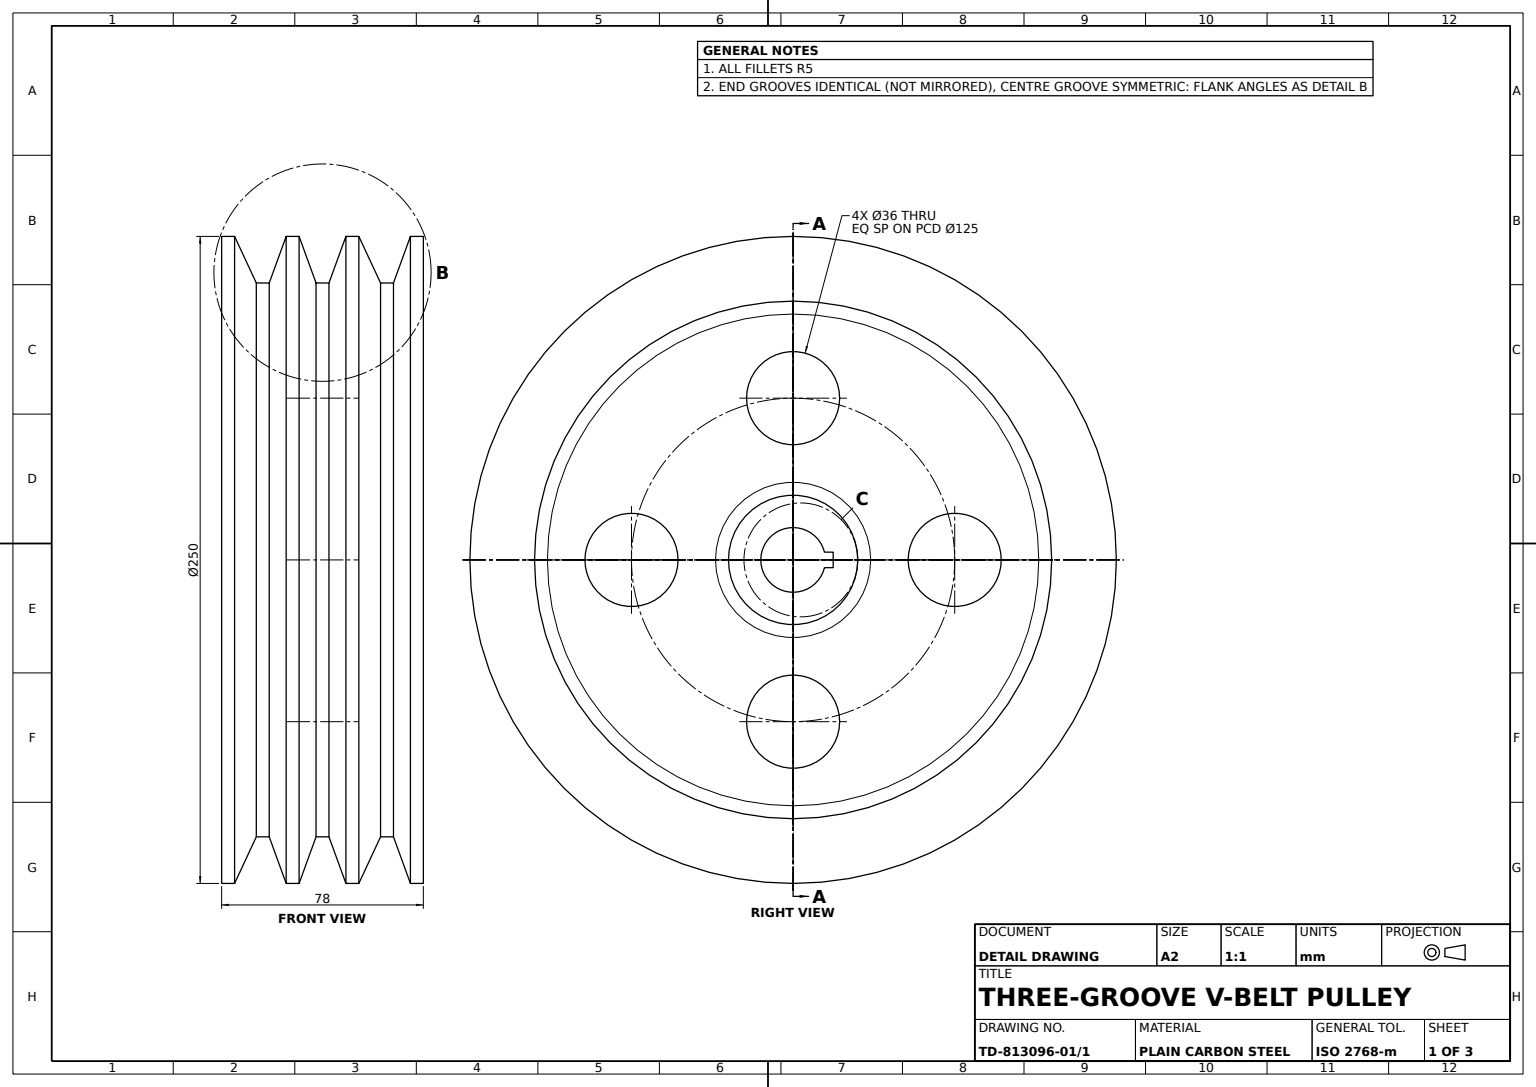
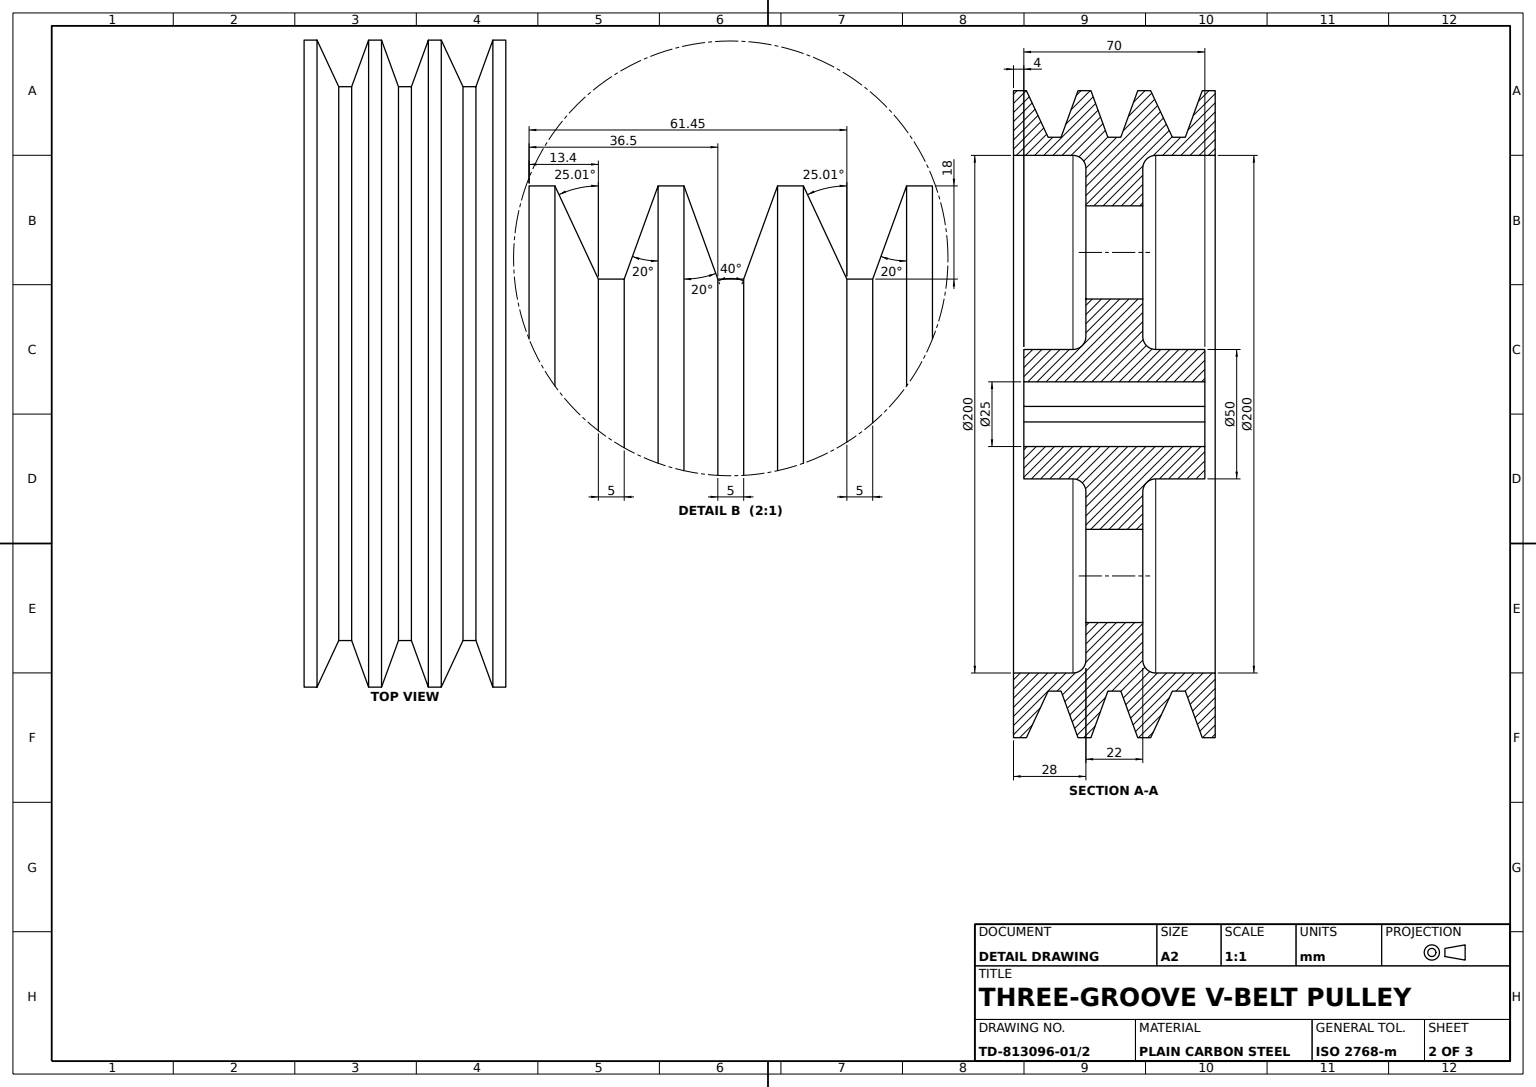
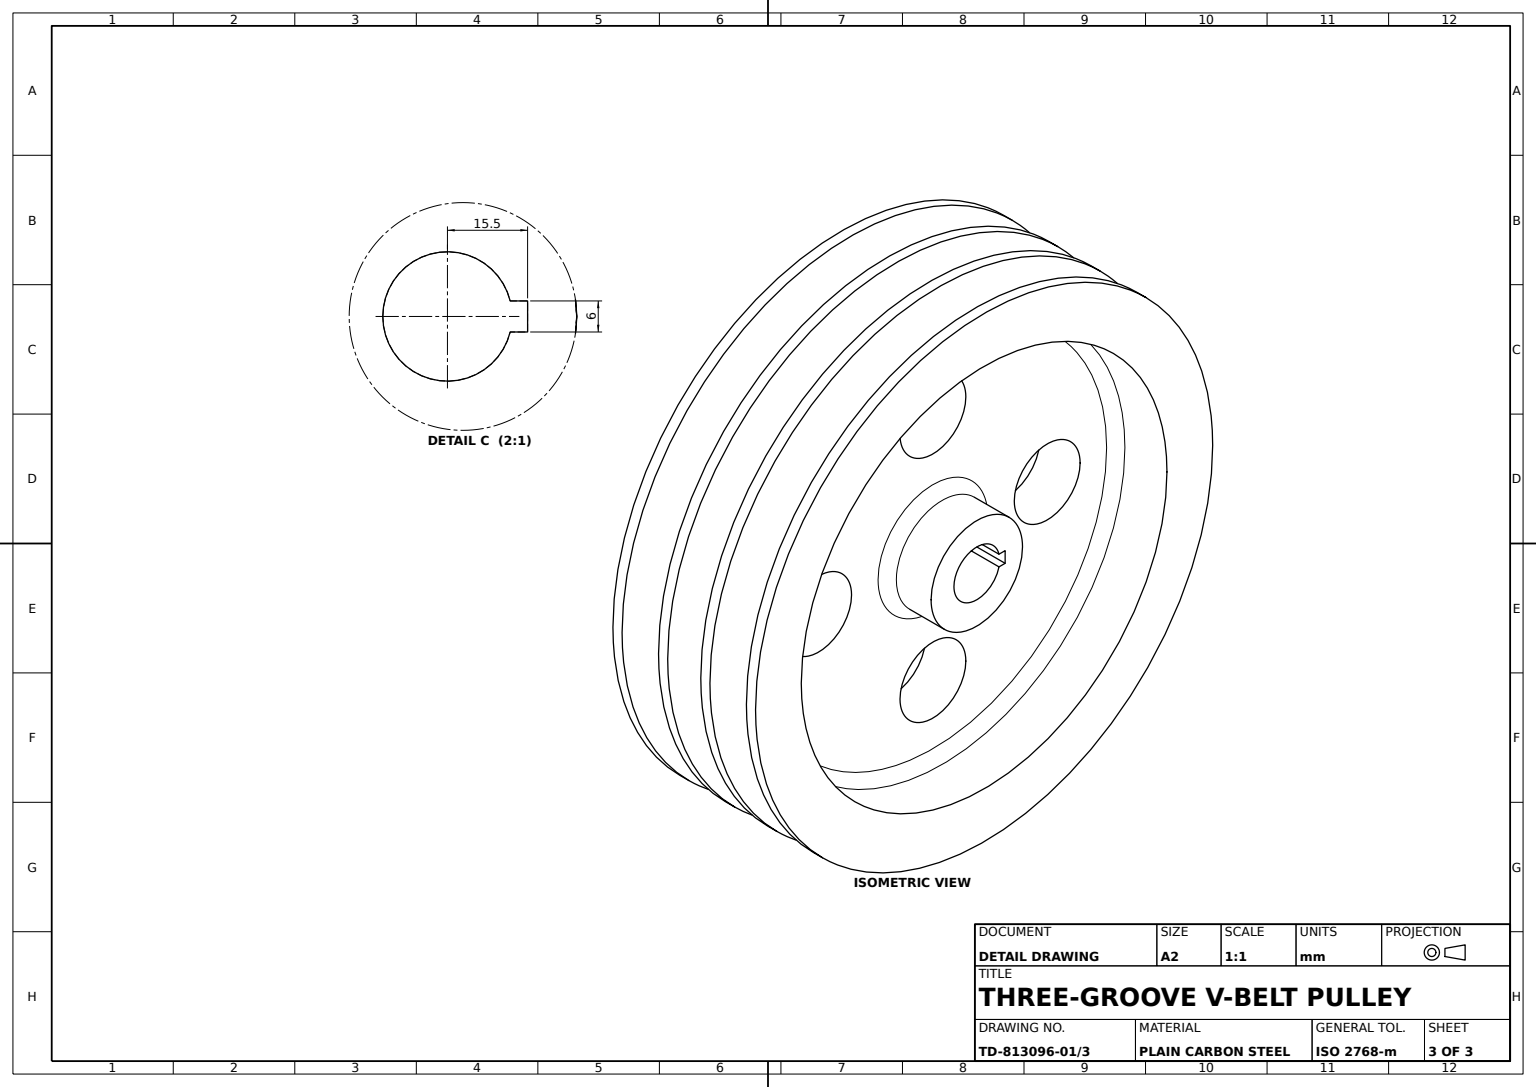
solid
v1 (35,3,-15.5)
v2 (35,3,-12.134661)
e1 v1 v2 LINE
v3 (-35,3,-12.134661)
e2 v3 v2 LINE
v4 (-35,3,-15.5)
e3 v4 v3 LINE
e4 v4 v1 LINE
face PLANE(AX(P(-45,3,-12.134661),D(0,1,0),D(0,0,1))) rev [e1 -e2 -e3 e4]
v5 (-11,0,80.5)
v6 (11,0,80.5)
e5 v5 v6 LINE
v7 (-11,0,44.5)
e6 v7 v5 CIRCLE(AX(P(-11,0,62.5),D(1,0,0),D(0,0,-1)),18)
v8 (11,0,44.5)
e7 v7 v8 LINE
e8 v6 v8 CIRCLE(AX(P(11,0,62.5),D(-1,0,0),D(0,0,1)),18)
face CYL(AX(P(-34,0,62.5),D(1,0,0),D(0,0,-1)),18) rev [-e5 -e6 e7 -e8]
v9 (-11,-62.5,18)
v10 (-11,-62.5,-18)
e9 v9 v10 CIRCLE(AX(P(-11,-62.5,0),D(1,0,0),D(0,0,-1)),18)
v11 (11,-62.5,18)
e10 v9 v11 LINE
v12 (11,-62.5,-18)
e11 v12 v11 CIRCLE(AX(P(11,-62.5,0),D(-1,0,0),D(0,0,1)),18)
e12 v10 v12 LINE
face CYL(AX(P(-34,-62.5,0),D(1,0,0),D(0,0,-1)),18) rev [-e9 e10 -e11 -e12]
v13 (35,0,25)
v14 (35,0,-25)
e13 v13 v14 CIRCLE(AX(P(35,0,0),D(-1,0,0),D(0,0,1)),25)
v15 (16,0,-25)
e14 v14 v15 LINE
v16 (16,0,25)
e15 v15 v16 CIRCLE(AX(P(16,0,0),D(1,0,0),D(0,0,1)),25)
e16 v13 v16 LINE
face CYL(AX(P(-52.075788,0,0),D(-1,0,0),D(0,0,1)),25) [e13 e14 e15 -e16]
v17 (-2.5,0,-107)
v18 (-2.5,0,107)
e17 v17 v18 CIRCLE(AX(P(-2.5,0,0),D(-1,0,0),D(0,0,1)),107)
v19 (-9.051464,0,125)
e18 v18 v19 LINE
v20 (-9.051464,0,-125)
e19 v20 v19 CIRCLE(AX(P(-9.051464,0,0),D(-1,0,0),D(0,0,1)),125)
e20 v17 v20 LINE
face CONE(AX(P(-2.5,0,0),D(-1,0,0),D(0,0,1)),107,1.221730476) [e17 e18 -e19 -e20]
v21 (-16,0,25)
v22 (-16,0,-25)
e21 v21 v22 CIRCLE(AX(P(-16,0,0),D(-1,0,0),D(0,0,-1)),25)
v23 (-35,0,-25)
e22 v22 v23 LINE
v24 (-35,0,25)
e23 v24 v23 CIRCLE(AX(P(-35,0,0),D(-1,0,0),D(0,0,1)),25)
e24 v21 v24 LINE
face CYL(AX(P(-52.075788,0,0),D(-1,0,0),D(0,0,1)),25) [e21 e22 -e23 -e24]
v25 (-16,0,-100)
v26 (-11,0,-95)
e25 v25 v26 CIRCLE(AX(P(-16,0,-95),D(0,-1,0),D(0,0,-1)),5)
v27 (-16,0,100)
e26 v27 v25 CIRCLE(AX(P(-16,0,0),D(1,0,0),D(0,0,-1)),100)
v28 (-11,0,95)
e27 v27 v28 CIRCLE(AX(P(-16,0,95),D(0,1,0),D(0,0,1)),5)
e28 v26 v28 CIRCLE(AX(P(-11,0,0),D(-1,0,0),D(0,0,-1)),95)
face TORUS(AX(P(-16,0,0),D(1,0,0),D(0,0,-1)),95,5) rev [-e25 -e26 e27 -e28]
v29 (-39,0,100)
v30 (-39,0,-100)
e29 v29 v30 CIRCLE(AX(P(-39,0,0),D(-1,0,0),D(0,0,1)),100)
e30 v25 v30 LINE
e31 v25 v27 CIRCLE(AX(P(-16,0,0),D(1,0,0),D(0,0,-1)),100)
e32 v27 v29 LINE
face CYL(AX(P(-52.075788,0,0),D(-1,0,0),D(0,0,1)),100) rev [e29 -e30 e31 e32]
v31 (39,0,-100)
v32 (39,0,100)
e33 v31 v32 CIRCLE(AX(P(39,0,0),D(-1,0,0),D(0,0,1)),100)
v33 (16,0,-100)
e34 v31 v33 LINE
v34 (16,0,100)
e35 v33 v34 CIRCLE(AX(P(16,0,0),D(-1,0,0),D(0,0,1)),100)
e36 v32 v34 LINE
face CYL(AX(P(-52.075788,0,0),D(-1,0,0),D(0,0,1)),100) rev [-e33 e34 e35 -e36]
v35 (2.5,0,107)
v36 (2.5,0,-107)
e37 v35 v36 CIRCLE(AX(P(2.5,0,0),D(-1,0,0),D(0,0,1)),107)
v37 (9.051464,0,125)
e38 v35 v37 LINE
v38 (9.051464,0,-125)
e39 v37 v38 CIRCLE(AX(P(9.051464,0,0),D(-1,0,0),D(0,0,1)),125)
e40 v36 v38 LINE
face CONE(AX(P(9.051464,0,0),D(1,0,0),D(0,0,-1)),125,1.221730476) [-e37 e38 e39 -e40]
v39 (22.448536,0,107)
v40 (14.051464,0,125)
e41 v39 v40 LINE
v41 (14.051464,0,-125)
e42 v41 v40 CIRCLE(AX(P(14.051464,0,0),D(-1,0,0),D(0,0,1)),125)
v42 (22.448536,0,-107)
e43 v42 v41 LINE
e44 v42 v39 CIRCLE(AX(P(22.448536,0,0),D(-1,0,0),D(0,0,1)),107)
face CONE(AX(P(22.448536,0,0),D(-1,0,0),D(0,0,1)),107,1.134302772) [e41 -e42 -e43 e44]
e45 v8 v6 CIRCLE(AX(P(11,0,62.5),D(-1,0,0),D(0,0,1)),18)
e46 v5 v7 CIRCLE(AX(P(-11,0,62.5),D(1,0,0),D(0,0,-1)),18)
face CYL(AX(P(-34,0,62.5),D(1,0,0),D(0,0,-1)),18) rev [e5 -e45 -e7 -e46]
v43 (-35,-3,-12.134661)
v44 (-35,0,12.5)
e47 v43 v44 CIRCLE(AX(P(-35,0,0),D(-1,0,0),D(0,0,1)),12.5)
v45 (35,0,12.5)
e48 v45 v44 LINE
v46 (35,-3,-12.134661)
e49 v46 v45 CIRCLE(AX(P(35,0,0),D(-1,0,0),D(0,0,1)),12.5)
e50 v43 v46 LINE
face CYL(AX(P(-52.075788,0,0),D(-1,0,0),D(0,0,1)),12.5) rev [e47 -e48 -e49 -e50]
v47 (27.448536,0,-107)
e51 v47 v42 LINE
v48 (27.448536,0,107)
e52 v47 v48 CIRCLE(AX(P(27.448536,0,0),D(-1,0,0),D(0,0,1)),107)
e53 v48 v39 LINE
face CYL(AX(P(-52.075788,0,0),D(-1,0,0),D(0,0,1)),107) [-e51 e52 e53 -e44]
e54 v19 v20 CIRCLE(AX(P(-9.051464,0,0),D(-1,0,0),D(0,0,1)),125)
e55 v18 v17 CIRCLE(AX(P(-2.5,0,0),D(-1,0,0),D(0,0,1)),107)
face CONE(AX(P(-2.5,0,0),D(-1,0,0),D(0,0,1)),107,1.221730476) [-e54 -e18 e55 e20]
e56 v40 v37 LINE
e57 v38 v37 CIRCLE(AX(P(9.051464,0,0),D(-1,0,0),D(0,0,1)),125)
e58 v41 v38 LINE
face CYL(AX(P(-52.075788,0,0),D(-1,0,0),D(0,0,1)),125) [e56 -e57 -e58 e42]
e59 v48 v47 CIRCLE(AX(P(27.448536,0,0),D(-1,0,0),D(0,0,1)),107)
e60 v39 v42 CIRCLE(AX(P(22.448536,0,0),D(-1,0,0),D(0,0,1)),107)
face CYL(AX(P(-52.075788,0,0),D(-1,0,0),D(0,0,1)),107) [e59 e51 -e60 -e53]
e61 v36 v17 LINE
e62 v35 v18 LINE
face CYL(AX(P(-52.075788,0,0),D(-1,0,0),D(0,0,1)),107) [e37 e61 -e55 -e62]
v49 (-35,-3,-15.5)
e63 v49 v4 LINE
v50 (35,-3,-15.5)
e64 v49 v50 LINE
e65 v50 v1 LINE
face PLANE(AX(P(-45,3,-15.5),D(0,0,-1),D(-1,0,0))) rev [-e63 e64 e65 -e4]
v51 (-11,0,-80.5)
v52 (-11,0,-44.5)
e66 v51 v52 CIRCLE(AX(P(-11,0,-62.5),D(1,0,0),D(0,0,-1)),18)
v53 (11,0,-80.5)
e67 v51 v53 LINE
v54 (11,0,-44.5)
e68 v54 v53 CIRCLE(AX(P(11,0,-62.5),D(-1,0,0),D(0,0,1)),18)
e69 v52 v54 LINE
face CYL(AX(P(-34,0,-62.5),D(1,0,0),D(0,0,-1)),18) rev [-e66 e67 -e68 -e69]
v55 (-25.602928,0,-107)
v56 (-25.602928,0,107)
e70 v55 v56 CIRCLE(AX(P(-25.602928,0,0),D(-1,0,0),D(0,0,1)),107)
v57 (-34,0,125)
e71 v56 v57 LINE
v58 (-34,0,-125)
e72 v58 v57 CIRCLE(AX(P(-34,0,0),D(-1,0,0),D(0,0,1)),125)
e73 v55 v58 LINE
face CONE(AX(P(-25.602928,0,0),D(-1,0,0),D(0,0,1)),107,1.134302772) [e70 e71 -e72 -e73]
v59 (-20.602928,0,-107)
v60 (-14.051464,0,-125)
e74 v59 v60 LINE
v61 (-20.602928,0,107)
e75 v61 v59 CIRCLE(AX(P(-20.602928,0,0),D(-1,0,0),D(0,0,1)),107)
v62 (-14.051464,0,125)
e76 v61 v62 LINE
e77 v62 v60 CIRCLE(AX(P(-14.051464,0,0),D(-1,0,0),D(0,0,1)),125)
face CONE(AX(P(-14.051464,0,0),D(1,0,0),D(0,0,-1)),125,1.221730476) [-e74 -e75 e76 e77]
e78 v23 v24 CIRCLE(AX(P(-35,0,0),D(-1,0,0),D(0,0,1)),25)
e79 v43 v49 LINE
e80 v44 v3 CIRCLE(AX(P(-35,0,0),D(-1,0,0),D(0,0,1)),12.5)
face PLANE(AX(P(-35,25,0),D(1,0,0),D(0,0,-1))) rev [e23 e78] [e79 e63 e3 -e80 -e47]
v63 (34,0,-125)
v64 (34,0,125)
e81 v63 v64 CIRCLE(AX(P(34,0,0),D(-1,0,0),D(0,0,1)),125)
v65 (39,0,-125)
e82 v65 v63 LINE
v66 (39,0,125)
e83 v65 v66 CIRCLE(AX(P(39,0,0),D(-1,0,0),D(0,0,1)),125)
e84 v66 v64 LINE
face CYL(AX(P(-52.075788,0,0),D(-1,0,0),D(0,0,1)),125) [-e81 -e82 e83 e84]
v67 (11,0,30)
e85 v67 v16 CIRCLE(AX(P(16,0,30),D(0,-1,0),D(0,0,-1)),5)
v68 (11,0,-30)
e86 v68 v67 CIRCLE(AX(P(11,0,0),D(-1,0,0),D(0,0,1)),30)
e87 v68 v15 CIRCLE(AX(P(16,0,-30),D(0,1,0),D(0,0,1)),5)
e88 v16 v15 CIRCLE(AX(P(16,0,0),D(1,0,0),D(0,0,1)),25)
face TORUS(AX(P(16,0,0),D(-1,0,0),D(0,0,1)),30,5) rev [-e85 -e86 e87 -e88]
v69 (11,0,-95)
e89 v33 v69 CIRCLE(AX(P(16,0,-95),D(0,1,0),D(0,0,1)),5)
v70 (11,0,95)
e90 v70 v69 CIRCLE(AX(P(11,0,0),D(1,0,0),D(0,0,1)),95)
e91 v34 v70 CIRCLE(AX(P(16,0,95),D(0,-1,0),D(0,0,-1)),5)
face TORUS(AX(P(16,0,0),D(-1,0,0),D(0,0,1)),95,5) rev [-e35 e89 -e90 -e91]
e92 v67 v68 CIRCLE(AX(P(11,0,0),D(-1,0,0),D(0,0,1)),30)
face TORUS(AX(P(16,0,0),D(-1,0,0),D(0,0,1)),30,5) rev [e85 -e15 -e87 -e92]
e93 v40 v41 CIRCLE(AX(P(14.051464,0,0),D(-1,0,0),D(0,0,1)),125)
face CYL(AX(P(-52.075788,0,0),D(-1,0,0),D(0,0,1)),125) [-e56 e93 e58 -e39]
v71 (-11,62.5,18)
v72 (11,62.5,18)
e94 v71 v72 LINE
v73 (11,62.5,-18)
e95 v73 v72 CIRCLE(AX(P(11,62.5,0),D(-1,0,0),D(0,0,1)),18)
v74 (-11,62.5,-18)
e96 v74 v73 LINE
e97 v71 v74 CIRCLE(AX(P(-11,62.5,0),D(1,0,0),D(0,0,-1)),18)
face CYL(AX(P(-34,62.5,0),D(1,0,0),D(0,0,-1)),18) rev [e94 -e95 -e96 -e97]
v75 (-39,0,-125)
e98 v58 v75 LINE
v76 (-39,0,125)
e99 v57 v76 LINE
e100 v75 v76 CIRCLE(AX(P(-39,0,0),D(-1,0,0),D(0,0,1)),125)
face CYL(AX(P(-52.075788,0,0),D(-1,0,0),D(0,0,1)),125) [-e98 e72 e99 -e100]
e101 v36 v35 CIRCLE(AX(P(2.5,0,0),D(-1,0,0),D(0,0,1)),107)
face CONE(AX(P(9.051464,0,0),D(1,0,0),D(0,0,-1)),125,1.221730476) [-e101 e40 e57 -e38]
e102 v69 v70 CIRCLE(AX(P(11,0,0),D(1,0,0),D(0,0,1)),95)
e103 v53 v54 CIRCLE(AX(P(11,0,-62.5),D(-1,0,0),D(0,0,1)),18)
e104 v11 v12 CIRCLE(AX(P(11,-62.5,0),D(-1,0,0),D(0,0,1)),18)
e105 v72 v73 CIRCLE(AX(P(11,62.5,0),D(-1,0,0),D(0,0,1)),18)
face PLANE(AX(P(11,25,0),D(-1,0,0),D(0,0,1))) rev [e102 e90] [e86 e92] [e103 e68] [e45 e8] [e11 e104] [e105 e95]
e106 v28 v26 CIRCLE(AX(P(-11,0,0),D(-1,0,0),D(0,0,-1)),95)
face TORUS(AX(P(-16,0,0),D(1,0,0),D(0,0,-1)),95,5) rev [-e31 e25 -e106 -e27]
e107 v10 v9 CIRCLE(AX(P(-11,-62.5,0),D(1,0,0),D(0,0,-1)),18)
face CYL(AX(P(-34,-62.5,0),D(1,0,0),D(0,0,-1)),18) rev [-e104 -e10 -e107 e12]
e108 v14 v13 CIRCLE(AX(P(35,0,0),D(-1,0,0),D(0,0,1)),25)
face CYL(AX(P(-52.075788,0,0),D(-1,0,0),D(0,0,1)),25) [-e14 e108 e16 e88]
e109 v20 v60 LINE
e110 v19 v62 LINE
face CYL(AX(P(-52.075788,0,0),D(-1,0,0),D(0,0,1)),125) [e54 e109 -e77 -e110]
e111 v60 v62 CIRCLE(AX(P(-14.051464,0,0),D(-1,0,0),D(0,0,1)),125)
e112 v59 v61 CIRCLE(AX(P(-20.602928,0,0),D(-1,0,0),D(0,0,1)),107)
face CONE(AX(P(-14.051464,0,0),D(1,0,0),D(0,0,-1)),125,1.221730476) [e74 e111 -e76 -e112]
e113 v22 v21 CIRCLE(AX(P(-16,0,0),D(-1,0,0),D(0,0,-1)),25)
face CYL(AX(P(-52.075788,0,0),D(-1,0,0),D(0,0,1)),25) [e113 e24 -e78 -e22]
e114 v30 v29 CIRCLE(AX(P(-39,0,0),D(-1,0,0),D(0,0,1)),100)
face CYL(AX(P(-52.075788,0,0),D(-1,0,0),D(0,0,1)),100) rev [e26 e30 e114 -e32]
e115 v34 v33 CIRCLE(AX(P(16,0,0),D(-1,0,0),D(0,0,1)),100)
face TORUS(AX(P(16,0,0),D(-1,0,0),D(0,0,1)),95,5) rev [-e102 -e89 -e115 e91]
e116 v52 v51 CIRCLE(AX(P(-11,0,-62.5),D(1,0,0),D(0,0,-1)),18)
face CYL(AX(P(-34,0,-62.5),D(1,0,0),D(0,0,-1)),18) rev [-e116 e69 -e103 -e67]
e117 v61 v56 LINE
e118 v59 v55 LINE
face CYL(AX(P(-52.075788,0,0),D(-1,0,0),D(0,0,1)),107) [e112 e117 -e70 -e118]
v77 (-11,0,-30)
v78 (-11,0,30)
e119 v77 v78 CIRCLE(AX(P(-11,0,0),D(1,0,0),D(0,0,-1)),30)
e120 v78 v77 CIRCLE(AX(P(-11,0,0),D(1,0,0),D(0,0,-1)),30)
e121 v74 v71 CIRCLE(AX(P(-11,62.5,0),D(1,0,0),D(0,0,-1)),18)
face PLANE(AX(P(-11,100,0),D(1,0,0),D(0,0,-1))) rev [e106 e28] [e66 e116] [e9 e107] [e119 e120] [e97 e121] [e46 e6]
face CYL(AX(P(-52.075788,0,0),D(-1,0,0),D(0,0,1)),107) [-e17 -e61 e101 e62]
face CONE(AX(P(22.448536,0,0),D(-1,0,0),D(0,0,1)),107,1.134302772) [-e41 e60 e43 -e93]
e122 v56 v55 CIRCLE(AX(P(-25.602928,0,0),D(-1,0,0),D(0,0,1)),107)
e123 v57 v58 CIRCLE(AX(P(-34,0,0),D(-1,0,0),D(0,0,1)),125)
face CONE(AX(P(-25.602928,0,0),D(-1,0,0),D(0,0,1)),107,1.134302772) [e122 e73 -e123 -e71]
e124 v32 v31 CIRCLE(AX(P(39,0,0),D(-1,0,0),D(0,0,1)),100)
face CYL(AX(P(-52.075788,0,0),D(-1,0,0),D(0,0,1)),100) rev [-e34 -e124 e36 e115]
e125 v66 v65 CIRCLE(AX(P(39,0,0),D(-1,0,0),D(0,0,1)),125)
e126 v64 v63 CIRCLE(AX(P(34,0,0),D(-1,0,0),D(0,0,1)),125)
face CYL(AX(P(-52.075788,0,0),D(-1,0,0),D(0,0,1)),125) [-e84 e125 e82 -e126]
e127 v46 v50 LINE
face PLANE(AX(P(-45,-3,-12.134661),D(0,-1,0),D(0,0,-1))) rev [e127 -e64 -e79 e50]
e128 v45 v2 CIRCLE(AX(P(35,0,0),D(-1,0,0),D(0,0,1)),12.5)
face PLANE(AX(P(35,12.5,0),D(-1,0,0),D(0,0,1))) rev [-e127 e49 e128 -e1 -e65] [-e108 -e13]
face PLANE(AX(P(39,100,0),D(-1,0,0),D(0,0,1))) rev [-e125 -e83] [e33 e124]
e129 v76 v75 CIRCLE(AX(P(-39,0,0),D(-1,0,0),D(0,0,1)),125)
face CYL(AX(P(-52.075788,0,0),D(-1,0,0),D(0,0,1)),125) [-e129 -e99 e123 e98]
e130 v47 v63 LINE
e131 v48 v64 LINE
face CONE(AX(P(34,0,0),D(1,0,0),D(0,0,-1)),125,1.221730476) [-e52 e130 e81 -e131]
face CYL(AX(P(-34,62.5,0),D(1,0,0),D(0,0,-1)),18) rev [-e121 e96 -e105 -e94]
face CONE(AX(P(34,0,0),D(1,0,0),D(0,0,-1)),125,1.221730476) [e131 e126 -e130 -e59]
e132 v77 v22 CIRCLE(AX(P(-16,0,-30),D(0,-1,0),D(0,0,-1)),5)
e133 v78 v21 CIRCLE(AX(P(-16,0,30),D(0,1,0),D(0,0,1)),5)
face TORUS(AX(P(-16,0,0),D(1,0,0),D(0,0,-1)),30,5) rev [-e132 -e120 e133 -e113]
face CYL(AX(P(-52.075788,0,0),D(-1,0,0),D(0,0,1)),12.5) rev [e2 -e128 e48 e80]
face TORUS(AX(P(-16,0,0),D(1,0,0),D(0,0,-1)),30,5) rev [-e119 e132 -e21 -e133]
face CYL(AX(P(-52.075788,0,0),D(-1,0,0),D(0,0,1)),107) [e75 e118 -e122 -e117]
face CYL(AX(P(-52.075788,0,0),D(-1,0,0),D(0,0,1)),125) [e110 -e111 -e109 e19]
face PLANE(AX(P(-39,125,0),D(1,0,0),D(0,0,-1))) rev [e100 e129] [-e29 -e114]
